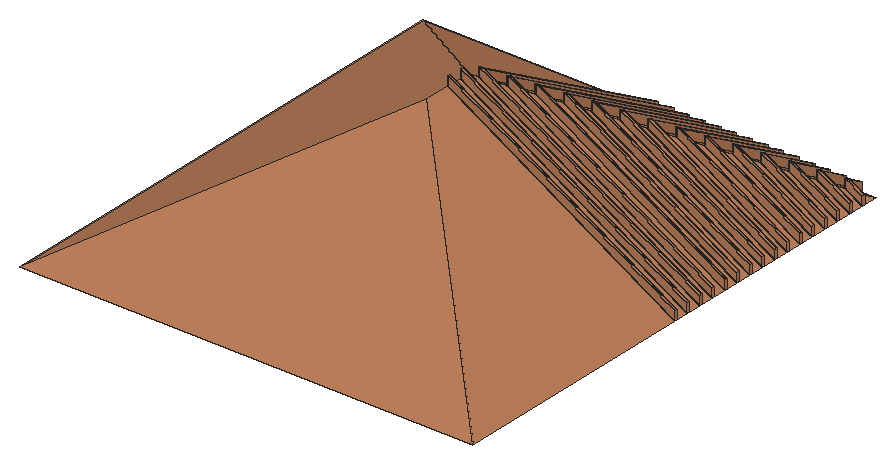
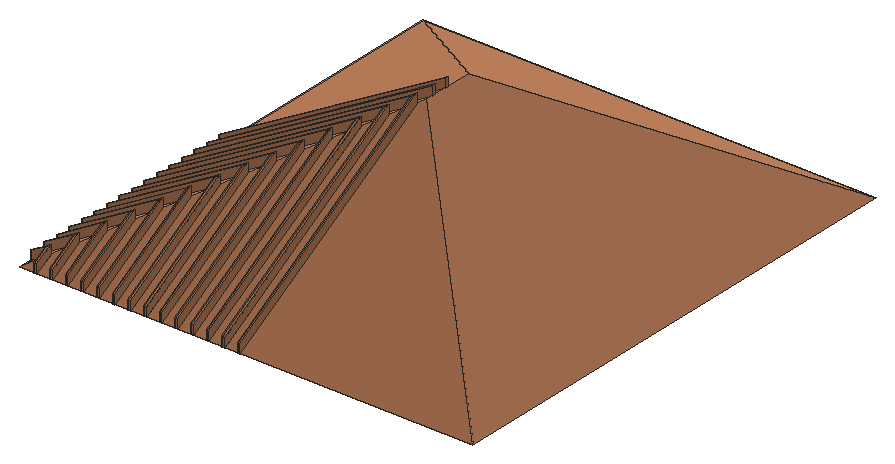
# SketchUp Ruby script. Lengths in millimetres.
U = 1.mm
M = Sketchup.active_model
def pt(a) = Geom::Point3d.new(a.map { |v| v * U })
def face(e, loops, mat)
  f = e.add_face(loops[0].map { |a| pt(a) })
  loops[1..].each { |l| e.add_face(l.map { |a| pt(a) }).erase! }
  f.material = f.back_material = mat if mat
  f
end
# faces: each face lists its corners as indices into pts; further lists are holes
def faces(e, pts, list, mat = nil) = list.each { |f| face(e, (f[0].is_a?(Array) ? f : [f]).map { |l| l.map { |i| pts[i] } }, mat) }
# xy, xz, yz: faces in a plane at the given z, y or x. An outline is a flat list of corners, or four numbers for a rectangle; further outlines are holes
def ring(l) = l.size == 4 ? [[l[0], l[1]], [l[2], l[1]], [l[2], l[3]], [l[0], l[3]]] : l.each_slice(2).to_a
def flat(e, list, mat, &to3) = list.each { |f| face(e, (f[0].is_a?(Array) ? f : [f]).map { |l| ring(l).map { |u, v| to3.(u, v) } }, mat) }
def xy(e, z, list, mat = nil) = flat(e, list, mat) { |x, y| [x, y, z] }
def xz(e, y, list, mat = nil) = flat(e, list, mat) { |x, z| [x, y, z] }
def yz(e, x, list, mat = nil) = flat(e, list, mat) { |y, z| [x, y, z] }
def lines(e, pts, list) = list.each { |a, b| e.add_line(pt(pts[a]), pt(pts[b])) }
# prism: a flat outline (further loops are holes) pulled along v
def prism(e, loops, v, mat = nil)
  f = face(e, loops, mat); d = Geom::Vector3d.new(v.map { |x| x * U })
  f.pushpull(f.normal.samedirection?(d) ? d.length : -d.length)
end
def box(e, o, s, mat = nil) = prism(e, [[o, [o[0] + s[0], o[1], o[2]], [o[0] + s[0], o[1] + s[1], o[2]], [o[0], o[1] + s[1], o[2]]]], [0, 0, s[2]], mat)
def at(x, y, z, deg = 0) = Geom::Transformation.translation(pt([x, y, z])) * Geom::Transformation.rotation(ORIGIN, Z_AXIS, deg.degrees)
def axes(o, x, y, z) = Geom::Transformation.new([*x, 0, *y, 0, *z, 0, *pt(o).to_a, 1])
def part(name) = M.definitions.add(name)
# library, detail: a bought-in or finely detailed component or shape, given as its bounding box
def library(name, o, s) = part(name).tap { |d| box(d.entities, o, s) }
def detail(e, o, s) = box(e.add_group.entities, o, s)
def put(e, d, t, mat = nil) = e.add_instance(d, t).tap { |i| i.material = mat if mat }
def group(e, t, mat = nil) = e.add_group.tap { |g| g.transformation = t; g.material = mat if mat }.entities
root = M.entities
M.materials.add("[Wood Veneer 02]").color = [190, 128, 91]
c1 = part("Group140\#1")
xy(c1.entities,0,[[-4901.1,-4575.5,-4960,-4524.5,0,-4524.5,0,-4575.5]])
xy(c1.entities,152,[[-4988.9,-4575.5,-87.8,-4575.5,-87.8,-4524.5,-5047.8,-4524.5]])
xz(c1.entities,-4575.5,[[-4901.1,0,0,0,-87.8,152,-4988.9,152]])
xz(c1.entities,-4524.5,[[-4960,0,-5047.8,152,-87.8,152,0,0]])
p = [[-4901.1,-4575.5,0],[-4988.9,-4575.5,152],[-5047.8,-4524.5,152],[-4960,-4524.5,0],[-87.8,-4575.5,152],[0,-4575.5,0],
  [0,-4524.5,0],[-87.8,-4524.5,152]]
faces(c1.entities,p,[[0,1,2,3],[4,5,6,7]])
c2 = part("Group138\#1")
xy(c2.entities,0,[[-4548.9,-4880.5,-4607.8,-4829.5,0,-4829.5,0,-4880.5]])
xy(c2.entities,152,[[-4636.7,-4880.5,-87.8,-4880.5,-87.8,-4829.5,-4695.6,-4829.5]])
xz(c2.entities,-4880.5,[[-4548.9,0,0,0,-87.8,152,-4636.7,152]])
xz(c2.entities,-4829.5,[[-4607.8,0,-4695.6,152,-87.8,152,0,0]])
p = [[-4695.6,-4829.5,152],[-4607.8,-4829.5,0],[-4548.9,-4880.5,0],[-4636.7,-4880.5,152],[0,-4829.5,0],[-87.8,-4829.5,152],
  [-87.8,-4880.5,152],[0,-4880.5,0]]
faces(c2.entities,p,[[0,1,2,3],[4,5,6,7]])
c3 = part("Group136\#1")
xy(c3.entities,0,[[-4196.8,-5185.5,-4255.6,-5134.5,0,-5134.5,0,-5185.5]])
xy(c3.entities,152,[[-4284.5,-5185.5,-87.8,-5185.5,-87.8,-5134.5,-4343.4,-5134.5]])
xz(c3.entities,-5185.5,[[-4196.8,0,0,0,-87.8,152,-4284.5,152]])
xz(c3.entities,-5134.5,[[-4255.6,0,-4343.4,152,-87.8,152,0,0]])
p = [[-4255.6,-5134.5,0],[-4196.8,-5185.5,0],[-4284.5,-5185.5,152],[-4343.4,-5134.5,152],[0,-5185.5,0],[0,-5134.5,0],
  [-87.8,-5134.5,152],[-87.8,-5185.5,152]]
faces(c3.entities,p,[[0,1,2,3],[4,5,6,7]])
c4 = part("Group134\#1")
xy(c4.entities,0,[[-3844.6,-5490.5,-3903.5,-5439.5,0,-5439.5,0,-5490.5]])
xy(c4.entities,152,[[-3932.3,-5490.5,-87.8,-5490.5,-87.8,-5439.5,-3991.2,-5439.5]])
xz(c4.entities,-5490.5,[[-3844.6,0,0,0,-87.8,152,-3932.3,152]])
xz(c4.entities,-5439.5,[[-3903.5,0,-3991.2,152,-87.8,152,0,0]])
p = [[-3932.3,-5490.5,152],[-3991.2,-5439.5,152],[-3903.5,-5439.5,0],[-3844.6,-5490.5,0],[-87.8,-5439.5,152],[-87.8,-5490.5,152],
  [0,-5490.5,0],[0,-5439.5,0]]
faces(c4.entities,p,[[0,1,2,3],[4,5,6,7]])
c5 = part("Group132\#1")
xy(c5.entities,0,[[-3492.4,-5795.5,-3551.3,-5744.5,0,-5744.5,0,-5795.5]])
xy(c5.entities,152,[[-3580.1,-5795.5,-87.8,-5795.5,-87.8,-5744.5,-3639,-5744.5]])
xz(c5.entities,-5795.5,[[-3492.4,0,0,0,-87.8,152,-3580.1,152]])
xz(c5.entities,-5744.5,[[-3551.3,0,-3639,152,-87.8,152,0,0]])
p = [[-3639,-5744.5,152],[-3551.3,-5744.5,0],[-3492.4,-5795.5,0],[-3580.1,-5795.5,152],[0,-5744.5,0],[-87.8,-5744.5,152],
  [-87.8,-5795.5,152],[0,-5795.5,0]]
faces(c5.entities,p,[[0,1,2,3],[4,5,6,7]])
c6 = part("Group130\#1")
xy(c6.entities,0,[[-3140.2,-6100.5,-3199.1,-6049.5,0,-6049.5,0,-6100.5]])
xy(c6.entities,152,[[-3228,-6100.5,-87.8,-6100.5,-87.8,-6049.5,-3286.9,-6049.5]])
xz(c6.entities,-6100.5,[[-3140.2,0,0,0,-87.8,152,-3228,152]])
xz(c6.entities,-6049.5,[[-3199.1,0,-3286.9,152,-87.8,152,0,0]])
p = [[-3286.9,-6049.5,152],[-3199.1,-6049.5,0],[-3140.2,-6100.5,0],[-3228,-6100.5,152],[0,-6049.5,0],[-87.8,-6049.5,152],
  [-87.8,-6100.5,152],[0,-6100.5,0]]
faces(c6.entities,p,[[0,1,2,3],[4,5,6,7]])
c7 = part("Group128\#1")
xy(c7.entities,0,[[-2788,-6405.5,-2846.9,-6354.5,0,-6354.5,0,-6405.5]])
xy(c7.entities,152,[[-2875.8,-6405.5,-87.8,-6405.5,-87.8,-6354.5,-2934.7,-6354.5]])
xz(c7.entities,-6405.5,[[-2788,0,0,0,-87.8,152,-2875.8,152]])
xz(c7.entities,-6354.5,[[-2846.9,0,-2934.7,152,-87.8,152,0,0]])
p = [[-2788,-6405.5,0],[-2875.8,-6405.5,152],[-2934.7,-6354.5,152],[-2846.9,-6354.5,0],[-87.8,-6405.5,152],[0,-6405.5,0],
  [0,-6354.5,0],[-87.8,-6354.5,152]]
faces(c7.entities,p,[[0,1,2,3],[4,5,6,7]])
c8 = part("Group93\#1")
prism(c8.entities,[[[-5180.2,-4851.4,152.4],[-88,-4851.4,152.4],[0,-4851.4,0],[-5092.2,-4851.4,0]]],[0,-50.8,0])
c9 = part("Group91\#1")
prism(c9.entities,[[[0,-4546.6,0],[-5092.2,-4546.6,0],[-5180.2,-4546.6,152.4],[-88,-4546.6,152.4]]],[0,-50.8,0])
c10 = part("Group89\#1")
xy(c10.entities,0,[[-4956.7,-4292.6,-4898,-4241.8,0,-4241.8,0,-4292.6]])
xy(c10.entities,152.4,[[-5044.7,-4292.6,-88,-4292.6,-88,-4241.8,-4986,-4241.8]])
xz(c10.entities,-4292.6,[[-4956.7,0,0,0,-88,152.4,-5044.7,152.4]])
xz(c10.entities,-4241.8,[[-4898,0,-4986,152.4,-88,152.4,0,0]])
p = [[-4898,-4241.8,0],[-4956.7,-4292.6,0],[-5044.7,-4292.6,152.4],[-4986,-4241.8,152.4],[0,-4292.6,0],[0,-4241.8,0],
  [-88,-4241.8,152.4],[-88,-4292.6,152.4]]
faces(c10.entities,p,[[0,1,2,3],[4,5,6,7]])
c11 = part("Group126\#1")
xy(c11.entities,0,[[-2435.8,-6710.5,-2494.7,-6659.5,0,-6659.5,0,-6710.5]])
xy(c11.entities,152,[[-2523.6,-6710.5,-87.8,-6710.5,-87.8,-6659.5,-2582.5,-6659.5]])
xz(c11.entities,-6710.5,[[-2435.8,0,0,0,-87.8,152,-2523.6,152]])
xz(c11.entities,-6659.5,[[-2494.7,0,-2582.5,152,-87.8,152,0,0]])
p = [[-2494.7,-6659.5,0],[-2435.8,-6710.5,0],[-2523.6,-6710.5,152],[-2582.5,-6659.5,152],[0,-6710.5,0],[0,-6659.5,0],
  [-87.8,-6659.5,152],[-87.8,-6710.5,152]]
faces(c11.entities,p,[[0,1,2,3],[4,5,6,7]])
c12 = part("Group87\#1")
xy(c12.entities,0,[[-4604.7,-3987.8,-4546.1,-3937,0,-3937,0,-3987.8]])
xy(c12.entities,152.4,[[-4692.7,-3987.8,-88,-3987.8,-88,-3937,-4634,-3937]])
xz(c12.entities,-3987.8,[[-4604.7,0,0,0,-88,152.4,-4692.7,152.4]])
xz(c12.entities,-3937,[[-4546.1,0,-4634,152.4,-88,152.4,0,0]])
p = [[-4546.1,-3937,0],[-4604.7,-3987.8,0],[-4692.7,-3987.8,152.4],[-4634,-3937,152.4],[0,-3987.8,0],[0,-3937,0],
  [-88,-3937,152.4],[-88,-3987.8,152.4]]
faces(c12.entities,p,[[0,1,2,3],[4,5,6,7]])
c13 = part("Group85\#1")
xy(c13.entities,0,[[-4252.8,-3683,-4194.1,-3632.2,0,-3632.2,0,-3683]])
xy(c13.entities,152.4,[[-4340.8,-3683,-88,-3683,-88,-3632.2,-4282.1,-3632.2]])
xz(c13.entities,-3683,[[-4252.8,0,0,0,-88,152.4,-4340.8,152.4]])
xz(c13.entities,-3632.2,[[-4194.1,0,-4282.1,152.4,-88,152.4,0,0]])
p = [[-4282.1,-3632.2,152.4],[-4194.1,-3632.2,0],[-4252.8,-3683,0],[-4340.8,-3683,152.4],[0,-3632.2,0],[-88,-3632.2,152.4],
  [-88,-3683,152.4],[0,-3683,0]]
faces(c13.entities,p,[[0,1,2,3],[4,5,6,7]])
c14 = part("Group124\#1")
xy(c14.entities,0,[[-2083.7,-7015.5,-2142.5,-6964.5,0,-6964.5,0,-7015.5]])
xy(c14.entities,152,[[-2171.4,-7015.5,-87.8,-7015.5,-87.8,-6964.5,-2230.3,-6964.5]])
xz(c14.entities,-7015.5,[[-2083.7,0,0,0,-87.8,152,-2171.4,152]])
xz(c14.entities,-6964.5,[[-2142.5,0,-2230.3,152,-87.8,152,0,0]])
p = [[-2171.4,-7015.5,152],[-2230.3,-6964.5,152],[-2142.5,-6964.5,0],[-2083.7,-7015.5,0],[-87.8,-6964.5,152],[-87.8,-7015.5,152],
  [0,-7015.5,0],[0,-6964.5,0]]
faces(c14.entities,p,[[0,1,2,3],[4,5,6,7]])
c15 = part("Group83\#1")
xy(c15.entities,0,[[-3900.8,-3378.2,-3842.2,-3327.4,0,-3327.4,0,-3378.2]])
xy(c15.entities,152.4,[[-3988.8,-3378.2,-88,-3378.2,-88,-3327.4,-3930.1,-3327.4]])
xz(c15.entities,-3378.2,[[-3900.8,0,0,0,-88,152.4,-3988.8,152.4]])
xz(c15.entities,-3327.4,[[-3842.2,0,-3930.1,152.4,-88,152.4,0,0]])
p = [[-3988.8,-3378.2,152.4],[-3930.1,-3327.4,152.4],[-3842.2,-3327.4,0],[-3900.8,-3378.2,0],[-88,-3327.4,152.4],[-88,-3378.2,152.4],
  [0,-3378.2,0],[0,-3327.4,0]]
faces(c15.entities,p,[[0,1,2,3],[4,5,6,7]])
c16 = part("Group81\#1")
xy(c16.entities,0,[[-3548.9,-3073.4,-3490.2,-3022.6,0,-3022.6,0,-3073.4]])
xy(c16.entities,152.4,[[-3636.8,-3073.4,-88,-3073.4,-88,-3022.6,-3578.2,-3022.6]])
xz(c16.entities,-3073.4,[[-3548.9,0,0,0,-88,152.4,-3636.8,152.4]])
xz(c16.entities,-3022.6,[[-3490.2,0,-3578.2,152.4,-88,152.4,0,0]])
p = [[-3548.9,-3073.4,0],[-3636.8,-3073.4,152.4],[-3578.2,-3022.6,152.4],[-3490.2,-3022.6,0],[-88,-3073.4,152.4],[0,-3073.4,0],
  [0,-3022.6,0],[-88,-3022.6,152.4]]
faces(c16.entities,p,[[0,1,2,3],[4,5,6,7]])
c17 = part("Group122\#1")
xy(c17.entities,0,[[-1731.5,-7320.5,-1790.4,-7269.5,0,-7269.5,0,-7320.5]])
xy(c17.entities,152,[[-1819.2,-7320.5,-87.8,-7320.5,-87.8,-7269.5,-1878.1,-7269.5]])
xz(c17.entities,-7320.5,[[-1731.5,0,0,0,-87.8,152,-1819.2,152]])
xz(c17.entities,-7269.5,[[-1790.4,0,-1878.1,152,-87.8,152,0,0]])
p = [[-1790.4,-7269.5,0],[-1731.5,-7320.5,0],[-1819.2,-7320.5,152],[-1878.1,-7269.5,152],[0,-7320.5,0],[0,-7269.5,0],
  [-87.8,-7269.5,152],[-87.8,-7320.5,152]]
faces(c17.entities,p,[[0,1,2,3],[4,5,6,7]])
c18 = part("Group79\#1")
xy(c18.entities,0,[[-3196.9,-2768.6,-3138.2,-2717.8,0,-2717.8,0,-2768.6]])
xy(c18.entities,152.4,[[-3284.9,-2768.6,-88,-2768.6,-88,-2717.8,-3226.2,-2717.8]])
xz(c18.entities,-2768.6,[[-3196.9,0,0,0,-88,152.4,-3284.9,152.4]])
xz(c18.entities,-2717.8,[[-3138.2,0,-3226.2,152.4,-88,152.4,0,0]])
p = [[-3226.2,-2717.8,152.4],[-3138.2,-2717.8,0],[-3196.9,-2768.6,0],[-3284.9,-2768.6,152.4],[0,-2717.8,0],[-88,-2717.8,152.4],
  [-88,-2768.6,152.4],[0,-2768.6,0]]
faces(c18.entities,p,[[0,1,2,3],[4,5,6,7]])
c19 = part("Group77\#1")
xy(c19.entities,0,[[-2845,-2463.8,-2786.3,-2413,0,-2413,0,-2463.8]])
xy(c19.entities,152.4,[[-2932.9,-2463.8,-88,-2463.8,-88,-2413,-2874.3,-2413]])
xz(c19.entities,-2463.8,[[-2845,0,0,0,-88,152.4,-2932.9,152.4]])
xz(c19.entities,-2413,[[-2786.3,0,-2874.3,152.4,-88,152.4,0,0]])
p = [[-2932.9,-2463.8,152.4],[-2874.3,-2413,152.4],[-2786.3,-2413,0],[-2845,-2463.8,0],[-88,-2413,152.4],[-88,-2463.8,152.4],
  [0,-2463.8,0],[0,-2413,0]]
faces(c19.entities,p,[[0,1,2,3],[4,5,6,7]])
c20 = part("Group120\#1")
xy(c20.entities,0,[[-1379.3,-7625.5,-1438.2,-7574.5,0,-7574.5,0,-7625.5]])
xy(c20.entities,152,[[-1467,-7625.5,-87.8,-7625.5,-87.8,-7574.5,-1525.9,-7574.5]])
xz(c20.entities,-7625.5,[[-1379.3,0,0,0,-87.8,152,-1467,152]])
xz(c20.entities,-7574.5,[[-1438.2,0,-1525.9,152,-87.8,152,0,0]])
p = [[-1379.3,-7625.5,0],[-1467,-7625.5,152],[-1525.9,-7574.5,152],[-1438.2,-7574.5,0],[-87.8,-7625.5,152],[0,-7625.5,0],
  [0,-7574.5,0],[-87.8,-7574.5,152]]
faces(c20.entities,p,[[0,1,2,3],[4,5,6,7]])
c21 = part("Group75\#1")
xy(c21.entities,0,[[-2493,-2159,-2434.3,-2108.2,0,-2108.2,0,-2159]])
xy(c21.entities,152.4,[[-2581,-2159,-88,-2159,-88,-2108.2,-2522.3,-2108.2]])
xz(c21.entities,-2159,[[-2493,0,0,0,-88,152.4,-2581,152.4]])
xz(c21.entities,-2108.2,[[-2434.3,0,-2522.3,152.4,-88,152.4,0,0]])
p = [[-2581,-2159,152.4],[-2522.3,-2108.2,152.4],[-2434.3,-2108.2,0],[-2493,-2159,0],[-88,-2108.2,152.4],[-88,-2159,152.4],
  [0,-2159,0],[0,-2108.2,0]]
faces(c21.entities,p,[[0,1,2,3],[4,5,6,7]])
c22 = part("Group73\#1")
xy(c22.entities,0,[[-2141,-1854.2,-2082.4,-1803.4,0,-1803.4,0,-1854.2]])
xy(c22.entities,152.4,[[-2229,-1854.2,-88,-1854.2,-88,-1803.4,-2170.4,-1803.4]])
xz(c22.entities,-1854.2,[[-2141,0,0,0,-88,152.4,-2229,152.4]])
xz(c22.entities,-1803.4,[[-2082.4,0,-2170.4,152.4,-88,152.4,0,0]])
p = [[-2141,-1854.2,0],[-2229,-1854.2,152.4],[-2170.4,-1803.4,152.4],[-2082.4,-1803.4,0],[-88,-1854.2,152.4],[0,-1854.2,0],
  [0,-1803.4,0],[-88,-1803.4,152.4]]
faces(c22.entities,p,[[0,1,2,3],[4,5,6,7]])
c23 = part("Group118\#1")
xy(c23.entities,0,[[-1027.1,-7930.5,-1086,-7879.5,0,-7879.5,0,-7930.5]])
xy(c23.entities,152,[[-1114.9,-7930.5,-87.8,-7930.5,-87.8,-7879.5,-1173.8,-7879.5]])
xz(c23.entities,-7930.5,[[-1027.1,0,0,0,-87.8,152,-1114.9,152]])
xz(c23.entities,-7879.5,[[-1086,0,-1173.8,152,-87.8,152,0,0]])
p = [[-1114.9,-7930.5,152],[-1173.8,-7879.5,152],[-1086,-7879.5,0],[-1027.1,-7930.5,0],[-87.8,-7879.5,152],[-87.8,-7930.5,152],
  [0,-7930.5,0],[0,-7879.5,0]]
faces(c23.entities,p,[[0,1,2,3],[4,5,6,7]])
c24 = part("Group71\#1")
xy(c24.entities,0,[[-1789.1,-1549.4,-1730.4,-1498.6,0,-1498.6,0,-1549.4]])
xy(c24.entities,152.4,[[-1877.1,-1549.4,-88,-1549.4,-88,-1498.6,-1818.4,-1498.6]])
xz(c24.entities,-1549.4,[[-1789.1,0,0,0,-88,152.4,-1877.1,152.4]])
xz(c24.entities,-1498.6,[[-1730.4,0,-1818.4,152.4,-88,152.4,0,0]])
p = [[-1730.4,-1498.6,0],[-1789.1,-1549.4,0],[-1877.1,-1549.4,152.4],[-1818.4,-1498.6,152.4],[0,-1549.4,0],[0,-1498.6,0],
  [-88,-1498.6,152.4],[-88,-1549.4,152.4]]
faces(c24.entities,p,[[0,1,2,3],[4,5,6,7]])
c25 = part("Group69\#1")
xy(c25.entities,0,[[-1437.1,-1244.6,-1378.5,-1193.8,0,-1193.8,0,-1244.6]])
xy(c25.entities,152.4,[[-1525.1,-1244.6,-88,-1244.6,-88,-1193.8,-1466.5,-1193.8]])
xz(c25.entities,-1244.6,[[-1437.1,0,0,0,-88,152.4,-1525.1,152.4]])
xz(c25.entities,-1193.8,[[-1378.5,0,-1466.5,152.4,-88,152.4,0,0]])
p = [[-1466.5,-1193.8,152.4],[-1378.5,-1193.8,0],[-1437.1,-1244.6,0],[-1525.1,-1244.6,152.4],[0,-1193.8,0],[-88,-1193.8,152.4],
  [-88,-1244.6,152.4],[0,-1244.6,0]]
faces(c25.entities,p,[[0,1,2,3],[4,5,6,7]])
c26 = part("Group116\#1")
xy(c26.entities,0,[[-674.9,-8235.5,-733.8,-8184.5,0,-8184.5,0,-8235.5]])
xy(c26.entities,152,[[-762.7,-8235.5,-87.8,-8235.5,-87.8,-8184.5,-821.6,-8184.5]])
xz(c26.entities,-8235.5,[[-674.9,0,0,0,-87.8,152,-762.7,152]])
xz(c26.entities,-8184.5,[[-733.8,0,-821.6,152,-87.8,152,0,0]])
p = [[-674.9,-8235.5,0],[-762.7,-8235.5,152],[-821.6,-8184.5,152],[-733.8,-8184.5,0],[-87.8,-8235.5,152],[0,-8235.5,0],
  [0,-8184.5,0],[-87.8,-8184.5,152]]
faces(c26.entities,p,[[0,1,2,3],[4,5,6,7]])
c27 = part("Group67\#1")
xy(c27.entities,0,[[-1085.2,-939.8,-1026.5,-889,0,-889,0,-939.8]])
xy(c27.entities,152.4,[[-1173.2,-939.8,-88,-939.8,-88,-889,-1114.5,-889]])
xz(c27.entities,-939.8,[[-1085.2,0,0,0,-88,152.4,-1173.2,152.4]])
xz(c27.entities,-889,[[-1026.5,0,-1114.5,152.4,-88,152.4,0,0]])
p = [[-1026.5,-889,0],[-1085.2,-939.8,0],[-1173.2,-939.8,152.4],[-1114.5,-889,152.4],[0,-939.8,0],[0,-889,0],
  [-88,-889,152.4],[-88,-939.8,152.4]]
faces(c27.entities,p,[[0,1,2,3],[4,5,6,7]])
c28 = part("Group65\#1")
xy(c28.entities,0,[[-733.2,-635,-674.6,-584.2,0,-584.2,0,-635]])
xy(c28.entities,152.4,[[-821.2,-635,-88,-635,-88,-584.2,-762.6,-584.2]])
xz(c28.entities,-635,[[-733.2,0,0,0,-88,152.4,-821.2,152.4]])
xz(c28.entities,-584.2,[[-674.6,0,-762.6,152.4,-88,152.4,0,0]])
p = [[-762.6,-584.2,152.4],[-674.6,-584.2,0],[-733.2,-635,0],[-821.2,-635,152.4],[0,-584.2,0],[-88,-584.2,152.4],
  [-88,-635,152.4],[0,-635,0]]
faces(c28.entities,p,[[0,1,2,3],[4,5,6,7]])
c29 = part("Group114\#1")
xy(c29.entities,0,[[-322.7,-8540.5,-381.6,-8489.5,0,-8489.5,0,-8540.5]])
xy(c29.entities,152,[[-410.5,-8540.5,-87.8,-8540.5,-87.8,-8489.5,-469.4,-8489.5]])
xz(c29.entities,-8540.5,[[-322.7,0,0,0,-87.8,152,-410.5,152]])
xz(c29.entities,-8489.5,[[-381.6,0,-469.4,152,-87.8,152,0,0]])
p = [[-322.7,-8540.5,0],[-410.5,-8540.5,152],[-469.4,-8489.5,152],[-381.6,-8489.5,0],[-87.8,-8540.5,152],[0,-8540.5,0],
  [0,-8489.5,0],[-87.8,-8489.5,152]]
faces(c29.entities,p,[[0,1,2,3],[4,5,6,7]])
c30 = part("Group63\#1")
xy(c30.entities,0,[[-381.3,-330.2,-322.6,-279.4,0,-279.4,0,-330.2]])
xy(c30.entities,152.4,[[-469.3,-330.2,-88,-330.2,-88,-279.4,-410.6,-279.4]])
xz(c30.entities,-330.2,[[-381.3,0,0,0,-88,152.4,-469.3,152.4]])
xz(c30.entities,-279.4,[[-322.6,0,-410.6,152.4,-88,152.4,0,0]])
p = [[-381.3,-330.2,0],[-469.3,-330.2,152.4],[-410.6,-279.4,152.4],[-322.6,-279.4,0],[-88,-330.2,152.4],[0,-330.2,0],
  [0,-279.4,0],[-88,-279.4,152.4]]
faces(c30.entities,p,[[0,1,2,3],[4,5,6,7]])
xy(root,3149.6,[[1303.3,1287,10123.3,11107]],"[Wood Veneer 02]")
p = [[10123.3,1287,3149.6],[5713.3,5697,5695.7],[1303.3,1287,3149.6],[5713.3,6697,5695.7],[1303.3,11107,3149.6],[10123.3,11107,3149.6]]
faces(root,p,[[0,1,2],[2,1,3,4],[5,3,1,0],[4,3,5]],"[Wood Veneer 02]")
put(root,c1,axes([1303.3,11107,3149.6],[0,0.86603,-0.5],[-1,0,0],[0,0.5,0.86603]),"[Wood Veneer 02]")
put(root,c2,axes([1303.3,11107,3149.6],[0,0.86603,-0.5],[-1,0,0],[0,0.5,0.86603]),"[Wood Veneer 02]")
put(root,c3,axes([1303.3,11107,3149.6],[0,0.86603,-0.5],[-1,0,0],[0,0.5,0.86603]),"[Wood Veneer 02]")
put(root,c4,axes([1303.3,11107,3149.6],[0,0.86603,-0.5],[-1,0,0],[0,0.5,0.86603]),"[Wood Veneer 02]")
put(root,c5,axes([1303.3,11107,3149.6],[0,0.86603,-0.5],[-1,0,0],[0,0.5,0.86603]),"[Wood Veneer 02]")
put(root,c6,axes([1303.3,11107,3149.6],[0,0.86603,-0.5],[-1,0,0],[0,0.5,0.86603]),"[Wood Veneer 02]")
put(root,c7,axes([1303.3,11107,3149.6],[0,0.86603,-0.5],[-1,0,0],[0,0.5,0.86603]),"[Wood Veneer 02]")
put(root,c8,axes([10123.3,11107,3149.6],[0.86603,0,-0.5],[0,1,0],[0.5,0,0.86603]),"[Wood Veneer 02]")
put(root,c9,axes([10123.3,11107,3149.6],[0.86603,0,-0.5],[0,1,0],[0.5,0,0.86603]),"[Wood Veneer 02]")
put(root,c10,axes([10123.3,11107,3149.6],[0.86603,0,-0.5],[0,1,0],[0.5,0,0.86603]),"[Wood Veneer 02]")
put(root,c11,axes([1303.3,11107,3149.6],[0,0.86603,-0.5],[-1,0,0],[0,0.5,0.86603]),"[Wood Veneer 02]")
put(root,c12,axes([10123.3,11107,3149.6],[0.86603,0,-0.5],[0,1,0],[0.5,0,0.86603]),"[Wood Veneer 02]")
put(root,c13,axes([10123.3,11107,3149.6],[0.86603,0,-0.5],[0,1,0],[0.5,0,0.86603]),"[Wood Veneer 02]")
put(root,c14,axes([1303.3,11107,3149.6],[0,0.86603,-0.5],[-1,0,0],[0,0.5,0.86603]),"[Wood Veneer 02]")
put(root,c15,axes([10123.3,11107,3149.6],[0.86603,0,-0.5],[0,1,0],[0.5,0,0.86603]),"[Wood Veneer 02]")
put(root,c16,axes([10123.3,11107,3149.6],[0.86603,0,-0.5],[0,1,0],[0.5,0,0.86603]),"[Wood Veneer 02]")
put(root,c17,axes([1303.3,11107,3149.6],[0,0.86603,-0.5],[-1,0,0],[0,0.5,0.86603]),"[Wood Veneer 02]")
put(root,c18,axes([10123.3,11107,3149.6],[0.86603,0,-0.5],[0,1,0],[0.5,0,0.86603]),"[Wood Veneer 02]")
put(root,c19,axes([10123.3,11107,3149.6],[0.86603,0,-0.5],[0,1,0],[0.5,0,0.86603]),"[Wood Veneer 02]")
put(root,c20,axes([1303.3,11107,3149.6],[0,0.86603,-0.5],[-1,0,0],[0,0.5,0.86603]),"[Wood Veneer 02]")
put(root,c21,axes([10123.3,11107,3149.6],[0.86603,0,-0.5],[0,1,0],[0.5,0,0.86603]),"[Wood Veneer 02]")
put(root,c22,axes([10123.3,11107,3149.6],[0.86603,0,-0.5],[0,1,0],[0.5,0,0.86603]),"[Wood Veneer 02]")
put(root,c23,axes([1303.3,11107,3149.6],[0,0.86603,-0.5],[-1,0,0],[0,0.5,0.86603]),"[Wood Veneer 02]")
put(root,c24,axes([10123.3,11107,3149.6],[0.86603,0,-0.5],[0,1,0],[0.5,0,0.86603]),"[Wood Veneer 02]")
put(root,c25,axes([10123.3,11107,3149.6],[0.86603,0,-0.5],[0,1,0],[0.5,0,0.86603]),"[Wood Veneer 02]")
put(root,c26,axes([1303.3,11107,3149.6],[0,0.86603,-0.5],[-1,0,0],[0,0.5,0.86603]),"[Wood Veneer 02]")
put(root,c27,axes([10123.3,11107,3149.6],[0.86603,0,-0.5],[0,1,0],[0.5,0,0.86603]),"[Wood Veneer 02]")
put(root,c28,axes([10123.3,11107,3149.6],[0.86603,0,-0.5],[0,1,0],[0.5,0,0.86603]),"[Wood Veneer 02]")
put(root,c29,axes([1303.3,11107,3149.6],[0,0.86603,-0.5],[-1,0,0],[0,0.5,0.86603]),"[Wood Veneer 02]")
put(root,c30,axes([10123.3,11107,3149.6],[0.86603,0,-0.5],[0,1,0],[0.5,0,0.86603]),"[Wood Veneer 02]")
